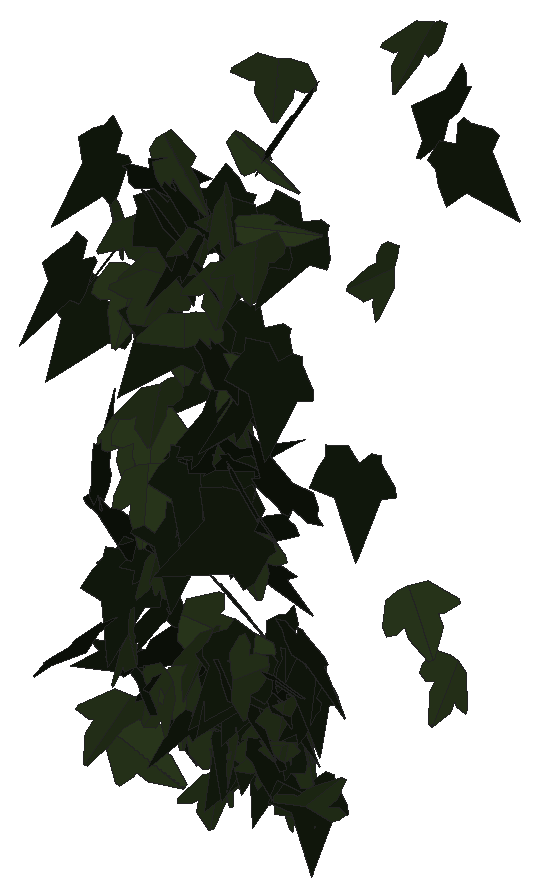
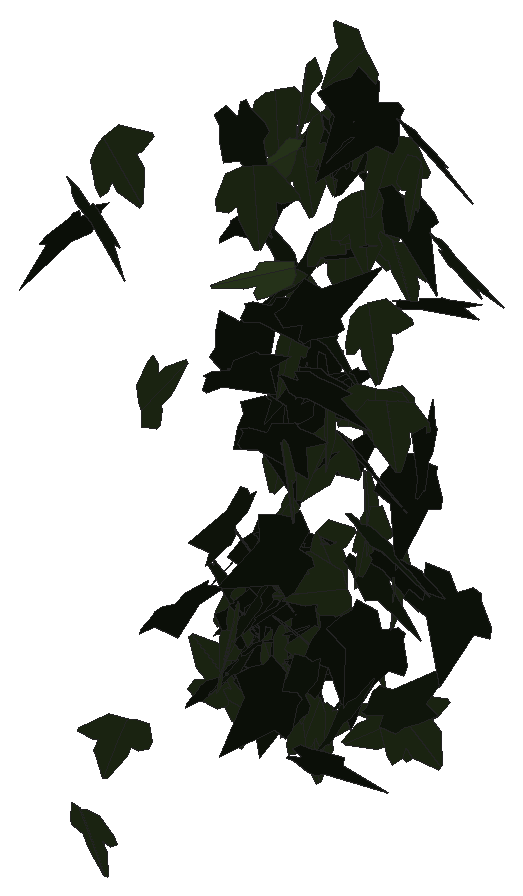
# SketchUp Ruby script. Lengths in inches.
U = 1.inch
M = Sketchup.active_model
def pt(a) = Geom::Point3d.new(a.map { |v| v * U })
def face(e, loops, mat)
  f = e.add_face(loops[0].map { |a| pt(a) })
  loops[1..].each { |l| e.add_face(l.map { |a| pt(a) }).erase! }
  f.material = f.back_material = mat if mat
  f
end
# faces: each face lists its corners as indices into pts; further lists are holes
def faces(e, pts, list, mat = nil) = list.each { |f| face(e, (f[0].is_a?(Array) ? f : [f]).map { |l| l.map { |i| pts[i] } }, mat) }
# xy, xz, yz: faces in a plane at the given z, y or x. An outline is a flat list of corners, or four numbers for a rectangle; further outlines are holes
def ring(l) = l.size == 4 ? [[l[0], l[1]], [l[2], l[1]], [l[2], l[3]], [l[0], l[3]]] : l.each_slice(2).to_a
def flat(e, list, mat, &to3) = list.each { |f| face(e, (f[0].is_a?(Array) ? f : [f]).map { |l| ring(l).map { |u, v| to3.(u, v) } }, mat) }
def xy(e, z, list, mat = nil) = flat(e, list, mat) { |x, y| [x, y, z] }
def xz(e, y, list, mat = nil) = flat(e, list, mat) { |x, z| [x, y, z] }
def yz(e, x, list, mat = nil) = flat(e, list, mat) { |y, z| [x, y, z] }
def lines(e, pts, list) = list.each { |a, b| e.add_line(pt(pts[a]), pt(pts[b])) }
# prism: a flat outline (further loops are holes) pulled along v
def prism(e, loops, v, mat = nil)
  f = face(e, loops, mat); d = Geom::Vector3d.new(v.map { |x| x * U })
  f.pushpull(f.normal.samedirection?(d) ? d.length : -d.length)
end
def box(e, o, s, mat = nil) = prism(e, [[o, [o[0] + s[0], o[1], o[2]], [o[0] + s[0], o[1] + s[1], o[2]], [o[0], o[1] + s[1], o[2]]]], [0, 0, s[2]], mat)
def at(x, y, z, deg = 0) = Geom::Transformation.translation(pt([x, y, z])) * Geom::Transformation.rotation(ORIGIN, Z_AXIS, deg.degrees)
def axes(o, x, y, z) = Geom::Transformation.new([*x, 0, *y, 0, *z, 0, *pt(o).to_a, 1])
def part(name) = M.definitions.add(name)
# library, detail: a bought-in or finely detailed component or shape, given as its bounding box
def library(name, o, s) = part(name).tap { |d| box(d.entities, o, s) }
def detail(e, o, s) = box(e.add_group.entities, o, s)
def put(e, d, t, mat = nil) = e.add_instance(d, t).tap { |i| i.material = mat if mat }
def group(e, t, mat = nil) = e.add_group.tap { |g| g.transformation = t; g.material = mat if mat }.entities
root = M.entities
M.materials.add("efeu1").color = [18, 25, 13]
M.materials.add("efeu2").color = [43, 57, 29]
c1 = part("ivyleaf_9")
p = [[1.54,2.16,1.25],[1.36,2.04,1.19],[-0.21,0.99,0.68],[-0.71,1.11,0.82],[-0.85,0.86,0.67],[-0.8,0.17,0.21],
  [-0.9,-0.01,0.1],[-0.67,-0.16,-0.02],[-0.08,-0.08,-0.05],[-0.03,-0.6,-0.4],[0.65,-0.88,-0.66],[0.83,-0.6,-0.49],
  [1.29,-0.42,-0.43],[1.8125,-0.07,-0.26],[1.21,0.44,0.15]]
faces(c1.entities,p,[[0,1,2,3,4,5,6,7,8,9,10,11,12,13,14]],"efeu1")
c2 = part("ivyleaf_10")
p = [[0,0.5,-0.03],[-0.0625,2.02,-0.43],[-0.19,2.01,-0.46],[-0.54,1.05,-0.29],[-0.52,0.625,-0.18],[-0.83,0.76,-0.28],
  [-1.16,0.64,-0.33],[-1.15,0.33,-0.24],[-0.77,-0.39,0.02],[-0.3,-0.51,0.16],[0.04,-0.48,0.23],[-0.02,2.01,-0.4375],
  [-0.06,2.01,-0.43],[0.04,-0.49,0.23],[0.67,-0.49,0.14],[1.38,0.36,-0.2],[1.375,0.51,-0.24],[0.81,0.65,-0.19],
  [0.62,0.59,-0.15],[0.6,1.09,-0.28],[0.5,1.23,-0.31]]
faces(c2.entities,p,[[0,1,2,3,4,5,6,7,8,9,10],[11,12,0,13,14,15,16,17,18,19,20]],"efeu2")
put(root,c1,axes([600.0625,124.96,296.27],[-1.1258,0.09096,-0.51064],[0.46874,-0.344,-1.09471],[-0.22205,-1.18736,0.27804]))
put(root,c1,axes([600.0625,128.48,278.48],[-1.04008,-0.32439,0.33875],[0.19691,-1.04991,-0.40082],[0.42569,-0.30692,1.01308]))
put(root,c2,axes([600.45,126.93,277.33],[-0.33858,-0.9713,0.66241],[-0.16587,-0.64297,-1.02758],[1.16391,-0.37418,0.04625]))
put(root,c1,axes([600.55,123.85,281.2],[0.1918,1.24661,0.32281],[-0.10913,0.34093,-1.25175],[-1.2831,0.15734,0.15472]))
put(root,c1,axes([600.59,125.74,294.42],[-0.97188,-0.72677,0.06942],[0.16072,-0.32573,-1.16001],[0.71217,-0.91829,0.35653]))
put(root,c1,axes([600.05,131.11,279.21],[0.15457,-0.96024,0.58902],[0.20428,-0.56079,-0.96783],[1.10783,0.23738,0.09628]))
put(root,c1,axes([600.91,125.08,287.33],[-0.01504,-0.29707,1.22609],[0.17569,1.21374,0.29623],[-1.24927,0.17427,0.0269]))
put(root,c1,axes([601.36,131.61,277.47],[-1.05124,-0.06468,0.41184],[-0.39785,-0.1781,-1.0435],[0.12454,-1.1149,0.1428]))
put(root,c1,axes([601.37,125.27,300.99],[-1.19771,0.20963,-0.20521],[0.19652,-0.06709,-1.2155],[-0.2178,-1.2133,0.03176]))
put(root,c1,axes([601.65,131.32,295.66],[-0.1245,0.06964,1.19227],[-1.02831,-0.6159,-0.0714],[0.6074,-1.02843,0.1235]))
put(root,c2,axes([601.4,125.22,299.21],[-0.94621,0.75703,0.10768],[-0.13627,0.00164,-1.2089],[-0.75241,-0.95231,0.08352]))
put(root,c1,axes([601.41,125.11,286.53],[0.94485,0.27481,-0.69298],[-0.68879,-0.10609,-0.98122],[-0.28514,1.16692,0.07399]))
put(root,c1,axes([601.26,126.44,283.38],[-0.91933,-0.4524,-0.5769],[0.58326,0.10923,-1.01514],[0.44415,-1.07983,0.139]))
put(root,c1,axes([601.99,125.01,297.8],[-0.5554,1.09572,-0.11493],[0.05736,-0.09978,-1.22843],[-1.10024,-0.55832,-0.00603]))
put(root,c1,axes([602.26,126.92,284.79],[-0.89756,0.71823,0.24274],[-0.30291,0.00511,-1.13517],[-0.695,-0.92979,0.18127]))
put(root,c2,axes([601.99,132,290.16],[0.67652,-0.79717,-0.55397],[-0.23972,0.51713,-1.0369],[0.94069,0.70508,0.13417]))
put(root,c1,axes([601.35,133.24,280.97],[1.12938,0.14662,-0.02922],[-0.02872,-0.00574,-1.13886],[-0.14672,1.12975,-0.00199]))
put(root,c2,axes([601.77,126.17,289.48],[1.05214,0.54316,-0.08048],[-0.17374,0.1643,-1.16246],[-0.52087,1.04235,0.22517]))
put(root,c1,axes([601.92,126.66,280.39],[0.40184,1.06673,0.28976],[0.10226,0.27112,-1.13991],[-1.10065,0.41465,-0.00012]))
put(root,c2,axes([601.96,125.39,295.89],[1.21827,-0.17816,-0.0046],[-0.00487,-0.00155,-1.23123],[0.17815,1.21828,-0.00223]))
put(root,c1,axes([601.4,131.79,280.22],[0.90304,-0.62188,0.31293],[0.28086,-0.14354,-1.09575],[0.63701,0.94489,0.0395]))
put(root,c2,axes([601.56,126.17,276.54],[-0.57692,-0.39967,-0.9265],[0.97988,0.03275,-0.62429],[0.24077,-1.09095,0.32069]))
put(root,c1,axes([603.02,126.12,282.59],[-0.87317,0.77355,-0.16763],[0.00566,-0.24349,-1.15307],[-0.79148,-0.85512,0.17669]))
put(root,c1,axes([602.5,132.36,291.09],[-0.89352,-0.75667,-0.1664],[0.13565,0.09728,-1.17079],[0.76279,-0.90366,0.0133]))
put(root,c1,axes([601.93,126.62,279.05],[0.87173,-0.77447,-0.11836],[-0.08206,0.08583,-1.16603],[0.77915,0.87554,0.00961]))
put(root,c2,axes([602.68,124.45,282.04],[0.31371,-0.91209,-0.72587],[-0.08588,0.73157,-0.95636],[1.1625,0.30018,0.12523]))
put(root,c2,axes([602.3,126.26,289.96],[1.07773,0.49298,0.08286],[0.08122,0.02163,-1.18505],[-0.49325,1.0807,-0.01408]))
put(root,c2,axes([602.9,132.85,301.73],[-1.03811,-0.62841,0.18081],[-0.14943,-0.1023,-1.21345],[0.63661,-1.04876,0.01002]))
put(root,c1,axes([602.65,134.35,294.61],[-0.65571,-0.9839,0.15873],[-0.04113,-0.16313,-1.18106],[0.99577,-0.65463,0.05574]))
put(root,c2,axes([602.63,126.3,284.59],[0.16698,-1.10158,-0.41446],[0.21403,0.44005,-1.08337],[1.15735,0.07756,0.26015]))
put(root,c1,axes([603.29,129.45,291.71],[-1.15826,-0.27085,0.07495],[-0.05996,-0.07239,-1.18815],[0.27455,-1.15842,0.05673]))
put(root,c1,axes([602.09,131.39,285.91],[1.11532,-0.02888,0.32476],[0.32602,0.08509,-1.11208],[0.00386,1.15852,0.08977]))
put(root,c1,axes([603.14,126.66,279.8],[0.19776,1.15058,-0.17519],[-0.0449,-0.17003,-1.16735],[-1.16297,0.20222,0.01527]))
put(root,c2,axes([603.07,125.89,285.76],[0.51524,-0.91984,-0.56841],[-0.13078,0.57201,-1.04421],[1.07335,0.51124,0.14563]))
put(root,c1,axes([603.02,131.47,295.86],[-0.85256,-0.8295,-0.15884],[0.16372,0.0591,-1.18738],[0.82855,-0.86522,0.07118]))
put(root,c1,axes([603.68,126.25,287.54],[-1.10977,0.39612,0.0108],[-0.00758,0.0109,-1.17833],[-0.3962,-1.10977,-0.00772]))
put(root,c2,axes([603.41,125.64,279.66],[0.83308,-0.60202,-0.56378],[-0.42936,0.36764,-1.02703],[0.70422,0.93633,0.04076]))
put(root,c2,axes([603.23,124.37,299.24],[-0.64923,-0.95307,-0.41336],[0.23347,0.34111,-1.15318],[1.01227,-0.68993,0.00086]))
put(root,c2,axes([603.55,125.55,297.26],[-0.59851,-1.06333,0.0383],[0.0111,-0.05018,-1.21972],[1.06396,-0.59763,0.03427]))
put(root,c2,axes([603.68,124.9,292.2],[-0.31876,-1.15959,0.0107],[-0.00488,-0.00976,-1.2026],[1.15963,-0.31879,-0.00212]))
put(root,c2,axes([603.46,124.65,288.66],[0.5989,1.02179,-0.16946],[-0.08028,-0.14937,-1.18436],[-1.03263,0.60422,-0.00621]))
put(root,c2,axes([603.98,124.72,296.78],[-0.78374,-0.8716,0.41452],[-0.22705,-0.35249,-1.17045],[0.93806,-0.81352,0.06303]))
put(root,c1,axes([603.52,124.87,301.32],[1.10066,0.5492,0.00749],[0.00509,0.00657,-1.23006],[-0.54923,1.10066,0.0036]))
put(root,c1,axes([604.31,125.36,295.01],[-0.87527,-0.80633,0.29196],[0.04216,-0.45713,-1.13612],[0.85652,-0.80148,0.35427]))
put(root,c2,axes([604.29,126.55,289.11],[0.42987,-1.04565,-0.35456],[0.07568,0.40749,-1.11001],[1.10153,0.38007,0.21462]))
put(root,c2,axes([604.21,127.69,276.83],[-0.94999,0.48872,-0.35756],[0.24014,-0.30662,-1.05711],[-0.5559,-0.96763,0.15438]))
put(root,c1,axes([604.17,125.74,286.89],[-0.20847,-1.1687,0.01594],[0.00325,-0.01677,-1.18713],[1.1688,-0.2084,0.00615]))
put(root,c1,axes([604.01,125.17,299.85],[0.22879,-1.15832,-0.36483],[-0.06574,0.35889,-1.18069],[1.21264,0.238,0.00482]))
put(root,c2,axes([603.7,130.37,296.53],[0.78034,-0.91535,-0.1047],[0.92126,0.7767,0.0759],[0.00981,-0.12894,1.20043]))
put(root,c2,axes([603.69,127.16,281.84],[0.23493,0.17688,1.12767],[0.92288,0.6481,-0.29392],[-0.67173,0.95227,-0.00942]))
put(root,c2,axes([604.47,127.03,279.24],[0.03324,0.95136,0.64808],[-0.09824,0.64833,-0.94669],[-1.14693,-0.02796,0.09987]))
put(root,c2,axes([604.73,127.08,275.79],[-0.34444,-1.06513,0.02709],[-0.01869,-0.02243,-1.11938],[1.06531,-0.34478,-0.01087]))
put(root,c1,axes([604.28,135.63,284.7],[-0.10868,-1.16397,-0.0813],[0.01989,0.0798,-1.16897],[1.16664,-0.10979,0.01235]))
put(root,c2,axes([604.25,125.73,280.25],[1.04511,-0.35637,0.40377],[0.38256,-0.12915,-1.1042],[0.37905,1.11293,0.00116]))
put(root,c2,axes([604.85,125.04,295.33],[-0.83356,-0.91265,0.03042],[0.10703,-0.13855,-1.22394],[0.90686,-0.82253,0.17242]))
put(root,c2,axes([604.65,126.42,287.27],[-1.05595,-0.4188,-0.37007],[0.36837,0.07338,-1.13415],[0.42029,-1.11651,0.06427]))
put(root,c1,axes([603.92,125.08,299.53],[0.95535,-0.91922,0.37954],[0.26664,-0.27026,-1.32573],[0.95808,0.99182,-0.0095]))
put(root,c1,axes([604.4375,127.39,278.94],[1.13268,-0.04449,-0.16027],[-0.15766,0.06435,-1.13209],[0.05301,1.14215,0.05754]))
put(root,c1,axes([605.4,125.38,280.1],[-1.01774,0.40526,-0.37422],[0.29982,-0.25279,-1.08916],[-0.46302,-1.05449,0.11728]))
put(root,c1,axes([605.69,127.37,279.625],[-1.10744,0.22953,0.00729],[-0.03773,-0.14646,-1.12084],[-0.22653,-1.09773,0.15107]))
put(root,c2,axes([604.3,129.19,300.64],[0.46726,-1.1039,0.24926],[1.07461,0.34824,-0.47221],[0.35486,0.39898,1.10179]))
put(root,c2,axes([605.24,125.4,278.79],[-0.09373,0.50593,1.05973],[-0.29932,1.01769,-0.51233],[-1.13551,-0.31002,0.04758]))
put(root,c2,axes([604.6875,128.02,277.06],[0.47268,-0.57451,-0.85162],[0.54844,-0.65154,0.74395],[-0.86864,-0.724,0.00629]))
put(root,c2,axes([605.37,125.53,282.37],[0.17206,-1.13453,0.29816],[0.01319,-0.29946,-1.14709],[1.17298,0.16978,-0.03083]))
put(root,c1,axes([605.72,124.56,299.52],[-1.01329,0.57898,-0.38317],[0.32954,-0.1956,-1.16703],[-0.6111,-1.06552,0.00602]))
put(root,c1,axes([605.08,125.69,289.1],[-0.26088,-1.17157,0.083],[0.02996,-0.09163,-1.19926],[1.17412,-0.25797,0.04905]))
put(root,c1,axes([606.02,125.29,291.74],[-0.90732,0.78913,0.0762],[-0.05266,0.05556,-1.20245],[-0.79105,-0.90882,-0.00735]))
put(root,c1,axes([605.82,130.02,302.1],[-0.63184,0.99784,-0.35188],[0.21725,-0.27876,-1.1806],[-1.03552,-0.66734,-0.03299]))
put(root,c1,axes([605.5625,126.93,278.53],[0.39913,1.04476,-0.16517],[-0.09994,-0.13849,-1.11756],[-1.05301,0.40916,0.04347]))
put(root,c2,axes([605.51,127.5,279.26],[0.05637,-1.14994,-0.01867],[-0.01415,0.01799,-1.15125],[1.15001,0.05659,-0.01325]))
put(root,c2,axes([605.46,135.8125,293.01],[-0.00334,-0.1723,-1.19313],[-0.19351,-1.17759,0.17059],[-1.18987,0.192,-0.0244]))
put(root,c1,axes([605.28,125.625,289.53],[0.96383,0.70001,-0.10289],[-0.10351,-0.03249,-1.19071],[-0.69992,0.96876,0.03442]))
put(root,c2,axes([604.7,124.36,302.71],[0.88544,-0.30802,0.84232],[0.89554,0.23909,-0.85395],[0.04892,1.19848,0.38684]))
put(root,c1,axes([605.24,127.57,278.49],[-0.17438,-1.12238,0.16708],[-0.0036,-0.16849,-1.13564],[1.13475,-0.17302,0.02207]))
put(root,c1,axes([604.85,124.78,300.71],[1.00589,-0.73274,-0.00047],[0.05257,0.07297,-1.24122],[0.73085,1.00324,0.08993]))
put(root,c2,axes([605.7,125.1,299.64],[-0.06265,-1.23346,0.02125],[-0.00143,-0.0212,-1.23505],[1.23364,-0.06266,-0.00035]))
put(root,c1,axes([605.75,127.73,277.91],[-0.83005,-0.77358,0.01734],[-0.01486,-0.00949,-1.13463],[0.77363,-0.83017,-0.00319]))
put(root,c1,axes([605.9,126.25,289.66],[-1.06376,-0.5304,-0.16639],[0.18628,-0.00163,-1.1857],[0.52374,-1.07669,0.08376]))
put(root,c1,axes([606.125,127.6875,276.92],[0.07127,0.98424,0.54845],[-0.13879,0.55303,-0.97442],[-1.11815,-0.00591,0.15591]))
put(root,c2,axes([606.04,127.9,278.61],[0.32809,-1.0767,0.15848],[0.03434,-0.1552,-1.12551],[1.08776,0.32965,-0.01227]))
put(root,c1,axes([605.93,126.79,280.24],[1.01702,0.42232,-0.42053],[-0.40471,-0.12119,-1.10048],[-0.4375,1.09384,0.04043]))
put(root,c1,axes([605.43,125.79,289.28],[0.57309,-0.03688,1.05806],[0.93171,0.58893,-0.48412],[-0.50277,1.04933,0.3089]))
put(root,c2,axes([606.2,126.28,291.38],[0.05195,-1.02424,-0.60939],[0.1153,0.61142,-1.01784],[1.18623,-0.01457,0.12562]))
put(root,c1,axes([605.98,127.47,280.51],[-0.34537,-1.0132,0.42149],[0.04954,-0.45582,-1.05512],[1.09625,-0.2986,0.18047]))
put(root,c2,axes([606.23,126.93,281.74],[1.12888,0.22971,-0.21732],[-0.20605,-0.07681,-1.15153],[-0.23987,1.14704,-0.03359]))
put(root,c2,axes([605.96,136.68,279.32],[0.71947,0.79738,0.35485],[0.196,0.30052,-1.07268],[-0.85048,0.7438,0.05299]))
put(root,c1,axes([606.02,127.48,279.05],[-0.37207,-1.06839,-0.03902],[0.24459,-0.04485,-1.10434],[1.04075,-0.37141,0.24559]))
put(root,c2,axes([606.47,138.14,275.91],[1.05258,-0.33927,-0.20892],[-0.19176,0.08593,-1.10567],[0.34925,1.06967,0.02256]))
put(root,c1,axes([605.875,125.43,294.38],[0.87922,-0.80287,-0.18138],[-0.10132,0.15781,-1.18969],[0.81684,0.88376,0.04766]))
put(root,c1,axes([606.5625,126.42,281.48],[-0.53438,-0.93945,0.40443],[-0.16046,-0.37364,-1.07997],[1.01014,-0.55634,0.0424]))
put(root,c2,axes([606.42,126,293.49],[1.19318,-0.16716,-0.00538],[-0.00672,-0.00925,-1.20479],[0.16711,1.19315,-0.0101]))
put(root,c2,axes([606.78,125.01,298.24],[-0.38959,-1.17178,0.09335],[0.0152,-0.10336,-1.23396],[1.1754,-0.38706,0.0469]))
put(root,c2,axes([606.89,136.14,303.1],[-0.14986,-1.13586,0.4883],[-0.1046,-0.47846,-1.14507],[1.23193,-0.17879,-0.03782]))
put(root,c2,axes([606.89,125.22,278.73],[0.67063,-0.87257,-0.43411],[-0.1587,0.42215,-1.0937],[0.96158,0.67822,0.12226]))
put(root,c1,axes([607.15,125.93,287.52],[0.19209,1.05919,-0.53623],[-0.19606,-0.50744,-1.07256],[-1.17089,0.25874,0.09163]))
put(root,c1,axes([607.16,125.87,282.25],[-1.03622,-0.52652,0.05533],[-0.02097,-0.0807,-1.16064],[0.52901,-1.03456,0.06238]))
put(root,c2,axes([606.91,125.94,286.77],[-1.14908,-0.30642,-0.11692],[0.13283,-0.04533,-1.1867],[0.29986,-1.15412,0.07765]))
put(root,c1,axes([606.35,125.99,281.17],[0.74974,-0.88297,0.03543],[0.00938,-0.03851,-1.1582],[0.88363,0.74959,-0.01777]))
put(root,c1,axes([607.58,125.35,287.74],[-0.81739,-0.63087,0.84082],[-0.65912,-0.52211,-1.0325],[0.81886,-1.05,0.00822]))
put(root,c1,axes([606.74,125.54,289.61],[1.04076,-0.36395,-0.46289],[-0.43842,0.14857,-1.10256],[0.39308,1.12933,-0.00413]))
put(root,c2,axes([606.89,124.66,301.03],[0.47041,-1.13561,-0.10487],[0.35383,0.25318,-1.15439],[1.08417,0.41011,0.42225]))
put(root,c1,axes([607.88,127.15,278.66],[-0.29435,-0.0008,1.12445],[-1.07685,-0.33441,-0.28213],[0.32371,-1.11319,0.08394]))
put(root,c1,axes([607.8,127.22,282.37],[-1.06576,0.4474,-0.10971],[0.11462,-0.01027,-1.15534],[-0.44617,-1.07135,-0.03474]))
put(root,c1,axes([607.3,125.79,281.6875],[0.95799,0.53116,-0.38862],[-0.46166,0.05321,-1.06534],[-0.46907,1.03245,0.25484]))
put(root,c1,axes([608.13,135.87,300.1875],[-0.55353,0.90753,0.65484],[-0.37042,0.5408,-1.06261],[-1.05604,-0.66539,0.02949]))
put(root,c2,axes([607.75,126.23,278.43],[-0.9982,-0.5519,-0.00445],[0.00182,0.00591,-1.14061],[0.55192,-0.99819,-0.00429]))
put(root,c1,axes([607.6,127,278.57],[-0.93117,-0.40484,-0.51126],[0.51783,0.08271,-1.00864],[0.3964,-1.05906,0.11666]))
put(root,c1,axes([608.2,124.83,293.81],[-1.02438,0.67503,-0.19723],[0.14965,-0.13126,-1.2265],[-0.68714,-1.03491,0.02691]))
put(root,c1,axes([607.04,127.36,280.39],[0.80728,-0.8004,-0.01432],[0.00125,0.02159,-1.1367],[0.80053,0.80712,0.01621]))
put(root,c1,axes([607.24,127.32,278.5625],[0.83265,-0.70813,-0.30782],[-0.20409,0.23475,-1.09212],[0.74468,0.85612,0.04486]))
put(root,c2,axes([607.89,126.75,279.85],[-0.23931,-1.15253,-0.03923],[0.01363,0.03724,-1.1771],[1.15312,-0.23963,0.00578]))
put(root,c2,axes([607.16,128.04,275.9],[-0.27692,0.10001,-1.09155],[0.83326,-0.71226,-0.27665],[-0.71215,-0.87227,0.10075]))
put(root,c2,axes([608.08,126.39,278.31],[-0.4914,-1.01638,0.13027],[-0.07429,-0.10876,-1.12877],[1.022,-0.4966,-0.01942]))
put(root,c1,axes([607.57,126,278.89],[0.78998,-0.46809,-0.71031],[-0.43957,0.60529,-0.88775],[0.7283,0.87305,0.23465]))
put(root,c2,axes([608.08,127.7,279.5625],[-0.88449,0.68941,0.18401],[-0.16794,0.0837,-1.12083],[-0.6935,-0.89954,0.03674]))
put(root,c2,axes([608.14,124.9,299.6],[-0.40855,-1.17096,-0.06937],[0.02817,0.06364,-1.24017],[1.17267,-0.40948,0.00563]))
put(root,c2,axes([608.24,127.81,277.19],[-0.45129,1.01792,-0.24488],[-0.0818,0.23156,1.11332],[1.04376,0.45826,-0.01863]))
put(root,c2,axes([608.08,124.1,282.54],[0.27483,-0.30312,-1.14992],[0.13057,1.18078,-0.28005],[1.18201,-0.05996,0.29831]))
put(root,c1,axes([609.06,127.15,280.63],[-0.95707,0.61294,-0.09726],[0.09353,-0.03425,-1.13632],[-0.61352,-0.96139,-0.02152]))
put(root,c1,axes([608.94,126.01,289.01],[0.74291,-0.51743,0.79441],[-0.66053,0.44148,0.90527],[-0.68008,-0.99403,-0.01146]))
put(root,c1,axes([608.52,127.76,276.67],[-0.03974,-1.14103,-0.01509],[0.00066,0.01508,-1.14172],[1.14113,-0.03975,0.00014]))
put(root,c1,axes([608.35,127.67,281.24],[0.24724,-1.0883,0.22054],[0.10168,-0.2028,-1.11477],[1.10576,0.26198,0.0532]))
put(root,c2,axes([608.66,126.97,275.96],[-0.48366,-0.87192,0.56299],[0.55111,0.31056,0.95444],[-0.87947,0.67411,0.28848]))
put(root,c1,axes([608.4,127.14,282.86],[0.72322,-0.87902,0.24827],[0.21237,-0.14617,-1.13617],[0.88837,0.75054,0.06949]))
put(root,c1,axes([608.9,125.22,295.07],[-0.19513,-1.19943,0.01731],[-0.01062,-0.01581,-1.21518],[1.19951,-0.19526,-0.00794]))
put(root,c1,axes([608.85,135.71,299.36],[0.53862,-0.77558,-0.82153],[-0.21767,0.82182,-0.91857],[1.10863,0.53817,0.21878]))
